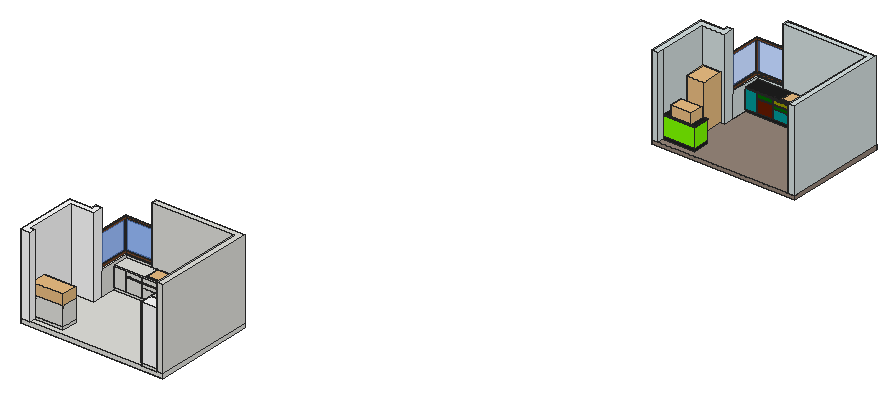
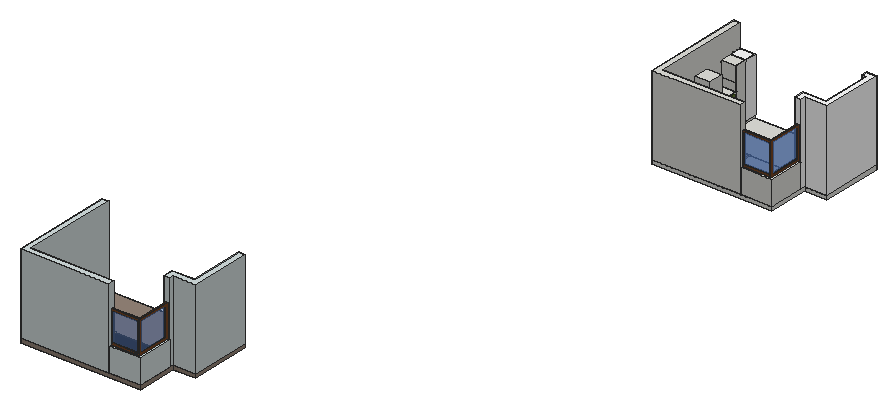
# SketchUp Ruby script. Lengths in inches.
U = 1.inch
M = Sketchup.active_model
def pt(a) = Geom::Point3d.new(a.map { |v| v * U })
def face(e, loops, mat)
  f = e.add_face(loops[0].map { |a| pt(a) })
  loops[1..].each { |l| e.add_face(l.map { |a| pt(a) }).erase! }
  f.material = f.back_material = mat if mat
  f
end
# faces: each face lists its corners as indices into pts; further lists are holes
def faces(e, pts, list, mat = nil) = list.each { |f| face(e, (f[0].is_a?(Array) ? f : [f]).map { |l| l.map { |i| pts[i] } }, mat) }
# xy, xz, yz: faces in a plane at the given z, y or x. An outline is a flat list of corners, or four numbers for a rectangle; further outlines are holes
def ring(l) = l.size == 4 ? [[l[0], l[1]], [l[2], l[1]], [l[2], l[3]], [l[0], l[3]]] : l.each_slice(2).to_a
def flat(e, list, mat, &to3) = list.each { |f| face(e, (f[0].is_a?(Array) ? f : [f]).map { |l| ring(l).map { |u, v| to3.(u, v) } }, mat) }
def xy(e, z, list, mat = nil) = flat(e, list, mat) { |x, y| [x, y, z] }
def xz(e, y, list, mat = nil) = flat(e, list, mat) { |x, z| [x, y, z] }
def yz(e, x, list, mat = nil) = flat(e, list, mat) { |y, z| [x, y, z] }
def lines(e, pts, list) = list.each { |a, b| e.add_line(pt(pts[a]), pt(pts[b])) }
# prism: a flat outline (further loops are holes) pulled along v
def prism(e, loops, v, mat = nil)
  f = face(e, loops, mat); d = Geom::Vector3d.new(v.map { |x| x * U })
  f.pushpull(f.normal.samedirection?(d) ? d.length : -d.length)
end
def box(e, o, s, mat = nil) = prism(e, [[o, [o[0] + s[0], o[1], o[2]], [o[0] + s[0], o[1] + s[1], o[2]], [o[0], o[1] + s[1], o[2]]]], [0, 0, s[2]], mat)
def at(x, y, z, deg = 0) = Geom::Transformation.translation(pt([x, y, z])) * Geom::Transformation.rotation(ORIGIN, Z_AXIS, deg.degrees)
def axes(o, x, y, z) = Geom::Transformation.new([*x, 0, *y, 0, *z, 0, *pt(o).to_a, 1])
def part(name) = M.definitions.add(name)
# library, detail: a bought-in or finely detailed component or shape, given as its bounding box
def library(name, o, s) = part(name).tap { |d| box(d.entities, o, s) }
def detail(e, o, s) = box(e.add_group.entities, o, s)
def put(e, d, t, mat = nil) = e.add_instance(d, t).tap { |i| i.material = mat if mat }
def group(e, t, mat = nil) = e.add_group.tap { |g| g.transformation = t; g.material = mat if mat }.entities
root = M.entities
M.materials.add("Carpaint Yellow 003 1.51cm").color = [255, 255, 255]
M.materials.add("T8600 Mosaic plaster 9142 31.87cm\#1").color = [255, 255, 255]
M.materials.add("[Blacktop New]").color = [30, 30, 30]
M.materials.add("[Carpet Berber Multi]").color = [151, 134, 122]
M.materials.add("[Color B08]").color = [102, 25, 0]
M.materials.add("[Color E07]").color = [153, 153, 0]
M.materials.add("[Color F05]").color = [127, 255, 0]
M.materials.add("[Color G08]").color = [0, 102, 0]
M.materials.add("[Color H07]").color = [0, 153, 153]
M.materials.add("[Translucent Glass Blue]").color = [100, 149, 237]
M.materials["[Translucent Glass Blue]"].alpha = 0.5
M.materials.add("[Translucent Glass Dark Green]").color = [62, 91, 5]
M.materials["[Translucent Glass Dark Green]"].alpha = 0.5
M.materials.add("[Wallpaper Dog Bone]").color = [213, 224, 224]
M.materials.add("[Wood Veneer 01]").color = [120, 70, 37]
c1 = library("Group\#83",[0,0,0],[47.24,22.83,19.96])
c2 = part("OuterShell")
prism(c2.entities,[[[0,0,0.08],[0,0,0.31],[0,0.59,0.31],[0,0.59,0.39],[0,0.79,0.39],[0,0.79,0],[0,0.59,0],[0,0.59,0.08]]],[0.39,0,0])
c3 = part("Cabinet pull handle")
put(c3.entities,c2,at(0,0,0))
put(c3.entities,c2,at(8.62,0,0))
g1 = group(c3.entities,at(0,0,0))
g2 = group(g1,at(0,0,0.2))
xy(g2,0,[[0.39,0.39,8.62,0.79]])
xy(g2,0.12,[[0.39,0.39,8.62,0.59]])
xy(g2,0.2,[[0.39,0.59,8.62,0.63],[0.39,0.63,8.62,0.79]])
xz(g2,0.39,[[0.39,0,8.62,0.12]])
xz(g2,0.59,[[0.39,0.12,8.62,0.2]])
xz(g2,0.79,[[0.39,0,8.62,0.2]])
yz(g2,0.39,[[0.39,0,0.39,0.12,0.59,0.12,0.59,0.2,0.79,0.2,0.79,0]])
yz(g2,8.62,[[0.39,0,0.79,0,0.79,0.2,0.59,0.2,0.59,0.12,0.39,0.12]])
g3 = group(g1,at(0,0,0.2))
xy(g3,-0.2,[[0.39,0.59,8.62,0.63],[0.39,0.63,8.62,0.79]])
xy(g3,-0.12,[[0.39,0.39,8.62,0.59]])
xy(g3,0,[[0.39,0.39,8.62,0.79]])
xz(g3,0.39,[[0.39,-0.12,8.62,0]])
xz(g3,0.59,[[0.39,-0.2,8.62,-0.12]])
xz(g3,0.79,[[0.39,-0.2,8.62,0]])
yz(g3,0.39,[[0.59,-0.2,0.79,-0.2,0.79,0,0.39,0,0.39,-0.12,0.59,-0.12]])
yz(g3,8.62,[[0.59,-0.2,0.59,-0.12,0.39,-0.12,0.39,0,0.79,0,0.79,-0.2]])
c4 = library("1-TABLE DE CUISSON CLC2\#1",[-11.42,-10.04,0],[22.84,20.08,1.26])
c5 = library("Fridge+large\#1",[35.74,-3.43,0],[31.11,25.36,66.28])
c6 = library("3-EVIER M80 CLC2",[-15.18,-9.87,-6.89],[30.32,19.69,21.27])
c7 = library("001",[-50.74,-66.02,15.67],[13.52,1.09,0.48])
c8 = part("Group\#8")
prism(c8.entities,[[[0,0,0],[0,90.79,0],[33.46,90.79,0],[33.46,151.42,0],[210.87,151.42,0],[210.87,0,0]]],[0,0,5.91])
xy(root,0,[[315.4375,884.73,362.68,907.57]])
xy(root,3.9375,[[315.4375,884.73,362.68,907.57]])
xy(root,31.5,[[315.4375,907.57,362.68,908.35]])
xy(root,33.07,[[[315.4375,884.73,362.68,908.35],[341.42,889.22,341.01,889.24,340.61,889.32,340.23,889.46,339.87,889.64,339.53,889.86,339.23,890.13,338.96,890.4375,338.74,890.77,338.56,891.14,338.43,891.52,338.35,891.92,338.32,892.32,338.32,902.2,338.38,902.6,338.5,902.98,338.66,903.35,338.86,903.7,339.11,904.01,339.4,904.29,339.72,904.54,340.07,904.74,340.4375,904.89,340.82,904.99,341.22,905.05,351.3125,905.05,351.68,905.01,352.04,904.93,352.39,904.8,352.72,904.63,353.02,904.43,353.3,904.18,353.55,903.91,353.76,903.6,353.93,903.28,354.0625,902.93,354.15,902.57,354.19,902.2,354.19,892.23,354.17,891.85,354.1,891.48,353.99,891.125,353.83,890.79,353.63,890.47,353.4,890.18,353.125,889.92,352.82,889.69,352.5,889.51,352.15,889.37,351.79,889.27,351.42,889.22],[329.55,889.23,329.21,889.27,328.87,889.34,328.55,889.46,328.24,889.625,327.95,889.82,327.69,890.05,327.46,890.31,327.27,890.59,327.11,890.9,326.99,891.23,326.91,891.5625,326.87,891.91,326.87,902.35,326.91,902.69,326.99,903.03,327.12,903.35,327.28,903.66,327.48,903.94,327.71,904.2,327.98,904.43,328.27,904.62,328.58,904.77,328.91,904.88,329.24,904.95,329.59,904.98,334.5,904.98,334.9,904.92,335.28,904.8,335.65,904.64,335.99,904.4375,336.3,904.1875,336.57,903.9,336.81,903.57,337,903.22,337.14,902.85,337.23,902.46,337.27,902.06,337.27,891.91,337.21,891.57,337.11,891.23,336.97,890.9,336.79,890.59,336.58,890.31,336.33,890.05,336.06,889.82,335.76,889.625,335.44,889.47,335.11,889.35,334.76,889.27,334.41,889.23]]],"[Blacktop New]")
xy(root,36,[[343.16,973.3125,345.66,975.8125],[343.16,975.8125,343.16,1023.93,386.3,1023.93,386.3,1022.68,344.41,1022.68,344.41,975.8125],[344.41,975.8125,344.41,1022.68,386.3,1022.68,386.3,1021.43,345.66,1021.43,345.66,975.8125]])
xy(root,38.5,[[343.16,975.8125,344.41,1021.43],[344.41,975.8125,345.66,1021.43],[345.66,1021.43,383.8,1022.68],[345.66,1022.68,383.8,1023.93]],"[Wood Veneer 01]")
xy(root,81.5,[[343.16,1021.43,345.66,1023.93]])
xy(root,81.5,[[343.16,975.8125,344.41,1021.43],[344.41,975.8125,345.66,1021.43],[345.66,1021.43,383.8,1022.68],[345.66,1022.68,383.8,1023.93]],"[Wood Veneer 01]")
xy(root,84,[[343.16,973.3125,344.41,973.3125,344.41,1022.68,386.3,1022.68,386.3,1023.93,343.16,1023.93],[344.41,973.3125,345.66,973.3125,345.66,1021.43,386.3,1021.43,386.3,1022.68,344.41,1022.68]])
xz(root,884.73,[[315.4375,0,362.68,3.9375],[315.4375,31.5,362.68,33.07]],"[Blacktop New]")
xz(root,884.73,[[315.4375,3.9375,362.68,31.5]],"[Color F05]")
xz(root,907.57,[[315.4375,0,362.68,3.9375]],"[Blacktop New]")
xz(root,907.57,[[315.4375,3.9375,362.68,31.5]],"[Color F05]")
xz(root,908.35,[[315.4375,31.5,362.68,33.07]],"[Blacktop New]")
xz(root,973.3125,[[343.16,36,344.41,84],[344.41,36,345.66,84]])
xz(root,975.8125,[[343.16,36,345.66,38.5]])
xz(root,975.8125,[[343.16,38.5,344.41,81.5],[344.41,38.5,345.66,81.5]],"[Wood Veneer 01]")
xz(root,1021.43,[[343.16,38.5,344.41,81.5]])
xz(root,1021.43,[[345.66,36,386.3,36,386.3,84,345.66,84,345.66,81.5,383.8,81.5,383.8,38.5,345.66,38.5],[344.41,38.5,345.66,81.5]],"[Wood Veneer 01]")
xz(root,1022.68,[[345.66,38.5,383.8,81.5]],"[Translucent Glass Blue]")
xz(root,1023.93,[[[343.16,36,386.3,84],[345.66,38.5,383.8,81.5]]],"[Wood Veneer 01]")
yz(root,315.4375,[[884.73,0,907.57,3.9375],[884.73,31.5,908.35,33.07]])
yz(root,343.16,[[[973.3125,36,1023.93,84],[975.8125,38.5,1021.43,81.5]]],"[Wood Veneer 01]")
yz(root,344.41,[[975.8125,38.5,1021.43,81.5]],"[Translucent Glass Blue]")
yz(root,345.66,[[973.3125,36,1021.43,36,1021.43,38.5,975.8125,38.5,975.8125,81.5,1021.43,81.5,1021.43,84,973.3125,84],[1021.43,38.5,1022.68,81.5],[1022.68,38.5,1023.93,81.5]],"[Wood Veneer 01]")
yz(root,362.68,[[884.73,0,907.57,3.9375],[884.73,31.5,908.35,33.07]],"[Blacktop New]")
yz(root,362.68,[[884.73,3.9375,907.57,31.5]],"[Color F05]")
yz(root,383.8,[[1021.43,38.5,1022.68,81.5],[1022.68,38.5,1023.93,81.5]],"[Wood Veneer 01]")
yz(root,386.3,[[1021.43,36,1022.68,84],[1022.68,36,1023.93,84]])
p = [[348.9,1018.2,31.5],[348.9,1018.2,33.07],[348.9,1018.2,0],[348.9,1018.2,3.9375],[508.35,1018.2,0],[484.73,1018.2,33.07],
  [338.07,895.54,45.01],[338.08,895.48,44.98],[337.87,895.23,44.88],[337.8,895.22,44.88],[337.66,895.25,44.89],[337.61,895.3,44.91],
  [338.07,895.41,44.95],[338.04,895.35,44.93],[338,895.3,44.91],[337.9375,895.25,44.89],[338,895.66,45.05],[338.04,895.61,45.03],
  [337.5625,895.35,44.93],[337.53,895.41,44.95],[337.73,895.73,45.08],[337.8,895.74,45.08],[337.52,895.48,44.98],[337.9375,895.7,45.07],
  [337.73,895.23,44.88],[337.61,895.66,45.05],[337.66,895.7,45.07],[337.87,895.73,45.08],[337.53,895.54,45.01],[337.5625,895.61,45.03]]
lines(root,p,[[0,1],[2,3],[4,2],[5,1],[6,7],[8,9],[10,11],[12,13],[14,15],[7,12],[16,17],[18,19],
  [17,6],[20,21],[19,22],[13,14],[11,18],[23,16],[9,24],[15,8],[24,10],[25,26],[21,27],[22,28],
  [28,29],[29,25],[27,23]])
g4 = group(root,at(0,92.51,0),"Carpaint Yellow 003 1.51cm")
g5 = group(g4,at(0,0,0))
prism(g5,[[[42.44,81.8125,0],[8.98,81.8125,0],[8.98,8.98,0],[14.76,8.98,0],[14.76,0,0],[0,0,0],[0,90.79,0],[33.46,90.79,0],[33.46,97.56,0],[42.44,97.56,0]]],[0,0,118.11])
g6 = group(root,at(8.98,101.49,0))
box(g6,[0,0,0],[47.24,22.83,3.9375])
g7 = group(root,at(8.98,101.49,3.9375))
xy(g7,0,[[0,0,47.24,22.83]])
xz(g7,0,[[0,0,47.24,27.56]])
xz(g7,22.83,[[0,0,47.24,27.56]])
yz(g7,0,[[0,0,22.83,27.56]])
yz(g7,47.24,[[0,0,22.83,27.56]])
put(root,c1,at(8.98,101.49,27.4))
g8 = group(root,at(37.85,192.57,38.58),"[Translucent Glass Blue]")
box(g8,[0,0,0],[0.2,45.62,43])
g9 = group(root,at(42.44,234.95,3.9375))
xy(g9,0,[[0,-22.83,17.72,0]])
xy(g9,0.06,[[0.06,-23.54,17.66,-22.83]])
xy(g9,27.5,[[0.06,-23.54,17.66,-22.83]])
xy(g9,27.56,[[0,-22.83,17.72,0]])
xz(g9,-23.54,[[0.06,0.06,17.66,27.5]])
xz(g9,-22.83,[[[0,0,17.72,27.56],[0.06,0.06,17.66,27.5]]])
xz(g9,0,[[0,0,17.72,27.56]])
yz(g9,0,[[-22.83,0,0,27.56]])
yz(g9,0.06,[[-23.54,0.06,-22.83,27.5]])
yz(g9,17.66,[[-23.54,0.06,-22.83,20.67],[-23.54,20.67,-22.83,27.5]])
yz(g9,17.72,[[-22.83,0,0,20.67],[-22.83,20.67,0,27.56]])
g10 = group(root,at(33.46,190.07,0))
prism(g10,[[[46.38,53.86,0],[46.38,44.88,0],[8.98,44.88,0],[8.98,0,0],[0,0,0],[0,53.86,0]]],[0,0,36.08])
g11 = group(root,at(36.7,190.07,36.08),"[Wood Veneer 01]")
xy(g11,0,[[0,0,0,50.62,43.14,50.62,43.14,48.12,2.5,48.12,2.5,0]])
xy(g11,2.5,[[0,2.5,2.5,48.12],[2.5,48.12,40.64,50.62]])
xy(g11,45.5,[[0,2.5,2.5,48.12],[2.5,48.12,40.64,50.62]])
xy(g11,48,[[0,0,2.5,0,2.5,48.12,43.14,48.12,43.14,50.62,0,50.62]])
xz(g11,0,[[0,0,2.5,48]])
xz(g11,2.5,[[0,2.5,2.5,45.5]])
xz(g11,48.12,[[2.5,0,43.14,0,43.14,48,2.5,48,2.5,45.5,40.64,45.5,40.64,2.5,2.5,2.5],[0,2.5,2.5,45.5]])
xz(g11,50.62,[[[0,0,43.14,48],[2.5,2.5,40.64,45.5]]])
yz(g11,0,[[[0,0,50.62,48],[2.5,2.5,48.12,45.5]]])
yz(g11,2.5,[[0,0,48.12,0,48.12,2.5,2.5,2.5,2.5,45.5,48.12,45.5,48.12,48,0,48],[48.12,2.5,50.62,45.5]])
yz(g11,40.64,[[48.12,2.5,50.62,45.5]])
yz(g11,43.14,[[48.12,0,50.62,48]])
g12 = group(root,at(39.2,239.44,38.58),"[Translucent Glass Blue]")
box(g12,[0,0,0],[38.14,0.2,43])
g13 = group(root,at(60.16,234.95,3.9375))
xy(g13,0,[[0,-22.83,23.62,0]])
xy(g13,0.06,[[0.06,-23.54,23.5625,-22.83]])
xy(g13,19.625,[[0.06,-23.54,23.5625,-22.83]])
xy(g13,20.67,[[0,-22.83,23.62,0]])
xz(g13,-23.54,[[0.06,0.06,23.5625,19.625]])
xz(g13,-22.83,[[[0,0,23.62,20.67],[0.06,0.06,23.5625,19.625]]])
xz(g13,0,[[0,0,23.62,20.67]])
yz(g13,0,[[-22.83,0,0,20.67]])
yz(g13,0.06,[[-23.54,0.06,-22.83,19.625]])
yz(g13,23.5625,[[-23.54,0.06,-22.83,13.78],[-23.54,13.78,-22.83,19.625]])
yz(g13,23.62,[[-22.83,0,0,13.78],[-22.83,13.78,0,20.67]])
g14 = group(root,at(60.16,234.95,24.61))
xy(g14,0,[[0,-22.83,23.62,0]])
xy(g14,0.06,[[0.06,-23.54,23.5625,-22.83]])
xy(g14,6.83,[[0.06,-23.54,23.5625,-22.83]])
xy(g14,6.89,[[0,-22.83,23.62,0]])
xz(g14,-23.54,[[0.06,0.06,23.5625,6.83]])
xz(g14,-22.83,[[[0,0,23.62,6.89],[0.06,0.06,23.5625,6.83]]])
xz(g14,0,[[0,0,23.62,6.89]])
yz(g14,0,[[-22.83,0,0,6.89]])
yz(g14,0.06,[[-23.54,0.06,-22.83,6.83]])
yz(g14,23.5625,[[-23.54,0.06,-22.83,6.83]])
yz(g14,23.62,[[-22.83,0,0,6.89]])
g15 = group(root,at(83.78,234.95,3.9375))
xy(g15,0,[[0,-22.83,35.43,0]])
xy(g15,0.06,[[0.06,-23.54,35.375,-22.83]])
xy(g15,13.72,[[0.06,-23.54,35.375,-22.83]])
xy(g15,13.78,[[0,-22.83,35.43,0]])
xz(g15,-23.54,[[0.06,0.06,35.375,13.72]])
xz(g15,-22.83,[[[0,0,35.43,13.78],[0.06,0.06,35.375,13.72]]])
xz(g15,0,[[0,0,35.43,13.78]])
yz(g15,0,[[-22.83,0,0,13.78]])
yz(g15,0.06,[[-23.54,0.06,-22.83,13.72]])
yz(g15,35.375,[[-23.54,0.06,-22.83,13.72]])
yz(g15,35.43,[[-22.83,0,0,13.78]])
g16 = group(root,at(83.78,234.95,17.72))
xy(g16,0,[[0,-22.83,35.43,0]])
xy(g16,0.06,[[0.06,-23.54,35.375,-22.83]])
xy(g16,5.85,[[0.06,-23.54,35.375,-22.83]])
xy(g16,6.89,[[0,-22.83,35.43,0]])
xz(g16,-23.54,[[0.06,0.06,35.375,5.85]])
xz(g16,-22.83,[[[0,0,35.43,6.89],[0.06,0.06,35.375,5.85]]])
xz(g16,0,[[0,0,35.43,6.89]])
yz(g16,0,[[-22.83,0,0,6.89]])
yz(g16,0.06,[[-23.54,0.06,-22.83,5.85]])
yz(g16,35.375,[[-23.54,0.06,-22.83,5.85]])
yz(g16,35.43,[[-22.83,0,0,6.89]])
g17 = group(root,at(83.78,234.95,24.61))
xy(g17,0,[[0,-22.83,35.43,0]])
xy(g17,0.06,[[0.06,-23.54,35.375,-22.83]])
xy(g17,6.83,[[0.06,-23.54,35.375,-22.83]])
xy(g17,6.89,[[0,-22.83,35.43,0]])
xz(g17,-23.54,[[0.06,0.06,35.375,6.83]])
xz(g17,-22.83,[[[0,0,35.43,6.89],[0.06,0.06,35.375,6.83]]])
xz(g17,0,[[0,0,35.43,6.89]])
yz(g17,0,[[-22.83,0,0,6.89]])
yz(g17,0.06,[[-23.54,0.06,-22.83,6.83]])
yz(g17,35.375,[[-23.54,0.06,-22.83,6.83]])
yz(g17,35.43,[[-22.83,0,0,6.89]])
put(root,c3,axes([60.22,212.12,23.48],[9.17031,0,0],[0,-1,0],[0,0,3]))
put(root,c4,at(102.04,222.98,33.07))
g18 = group(root,at(0,92.51,-6))
prism(g18,[[[33.46,151.42,0],[210.87,151.42,0],[210.87,0,0],[0,0,0],[0,90.79,0],[33.46,90.79,0]]],[0,0,6])
g19 = group(root,at(42.44,234.95,0))
prism(g19,[[[41.34,0,3.9375],[76.77,0,3.9375],[100.39,0,3.9375],[124.02,0,3.9375],[136.61,0,3.9375],[159.45,0,3.9375],[159.45,0,0],[0,0,0],[0,0,3.9375],[17.72,0,3.9375]]],[0,-22.83,0])
g20 = group(root,at(42.44,234.95,31.5))
box(g20,[0,-23.62,0],[159.45,23.62,1.57])
g21 = group(root,at(119.21,234.95,3.9375))
xy(g21,0,[[0,-22.83,23.62,0]])
xy(g21,0.06,[[0.06,-23.54,23.5625,-22.83]])
xy(g21,19.625,[[0.06,-23.54,23.5625,-22.83]])
xy(g21,20.67,[[0,-22.83,23.62,0]])
xz(g21,-23.54,[[0.06,0.06,23.5625,19.625]])
xz(g21,-22.83,[[[0,0,23.62,20.67],[0.06,0.06,23.5625,19.625]]])
xz(g21,0,[[0,0,23.62,20.67]])
yz(g21,0,[[-22.83,0,0,13.78],[-22.83,13.78,0,20.67]])
yz(g21,0.06,[[-23.54,0.06,-22.83,13.78],[-23.54,13.78,-22.83,19.625]])
yz(g21,23.5625,[[-23.54,0.06,-22.83,19.625]])
yz(g21,23.62,[[-22.83,0,0,20.67]])
g22 = group(root,at(119.21,234.95,24.61))
xy(g22,0,[[0,-22.83,23.62,0]])
xy(g22,0.06,[[0.06,-23.54,23.5625,-22.83]])
xy(g22,6.83,[[0.06,-23.54,23.5625,-22.83]])
xy(g22,6.89,[[0,-22.83,23.62,0]])
xz(g22,-23.54,[[0.06,0.06,23.5625,6.83]])
xz(g22,-22.83,[[[0,0,23.62,6.89],[0.06,0.06,23.5625,6.83]]])
xz(g22,0,[[0,0,23.62,6.89]])
yz(g22,0,[[-22.83,0,0,6.89]])
yz(g22,0.06,[[-23.54,0.06,-22.83,6.83]])
yz(g22,23.5625,[[-23.54,0.06,-22.83,6.83]])
yz(g22,23.62,[[-22.83,0,0,6.89]])
g23 = group(root,at(79.84,92.51,0))
g24 = group(g23,at(0,0,0))
prism(g24,[[[131.02,0,0],[122.05,0,0],[122.05,142.44,0],[0,142.44,0],[0,151.42,0],[131.02,151.42,0]]],[0,0,118.11])
g25 = group(root,at(142.83,234.95,3.9375))
xy(g25,0,[[0,-22.83,23.62,0]])
xy(g25,0.06,[[0.06,-23.54,23.5625,-22.83]])
xy(g25,27.5,[[0.06,-23.54,23.5625,-22.83]])
xy(g25,27.56,[[0,-22.83,23.62,0]])
xz(g25,-23.54,[[0.06,0.06,23.5625,27.5]])
xz(g25,-22.83,[[[0,0,23.62,27.56],[0.06,0.06,23.5625,27.5]]])
xz(g25,0,[[0,0,23.62,27.56]])
yz(g25,0,[[-22.83,0,0,20.67],[-22.83,20.67,0,27.56]])
yz(g25,0.06,[[-23.54,0.06,-22.83,27.5]])
yz(g25,23.5625,[[-23.54,0.06,-22.83,27.5]])
yz(g25,23.62,[[-22.83,0,0,27.56]])
g26 = group(root,at(166.46,234.95,3.9375))
xy(g26,0,[[0,-22.83,12.6,0]])
xy(g26,0.06,[[0.06,-23.54,10.96,-22.83]])
xy(g26,27.5,[[0.06,-23.54,10.96,-22.83]])
xy(g26,27.56,[[0,-22.83,12.6,0]])
xz(g26,-23.54,[[0.06,0.06,10.96,27.5]])
xz(g26,-22.83,[[[0,0,12.6,27.56],[0.06,0.06,12.54,27.5]],[10.96,0.06,11.02,27.5],[11.02,0.06,12.54,27.5]])
xz(g26,0,[[0,0,12.6,27.56]])
yz(g26,0,[[-22.83,0,0,27.56]])
yz(g26,0.06,[[-23.54,0.06,-22.83,27.5]])
yz(g26,10.96,[[-23.54,0.06,-22.83,27.5]])
yz(g26,12.6,[[-22.83,0,0,27.56]])
g27 = group(root,at(201.89,234.95,31.5))
prism(g27,[[[-23.62,-22.83,0],[-23.62,-35.43,0],[-23.62,-61.02,0],[-23.62,-81.42,0],[-23.62,-81.42,1.57],[-23.62,-57.8,1.57],[-23.62,0,1.57],[-23.62,0,0]]],[23.62,0,0])
g28 = group(root,at(201.89,153.54,3.9375))
xy(g28,0,[[-22.83,-25.59,0,0]])
xy(g28,0.06,[[-23.54,-25.53,-22.83,-0.06]])
xy(g28,22.22,[[-23.54,-25.53,-22.83,-0.06]])
xy(g28,22.28,[[-22.83,-25.59,0,0]])
xz(g28,-25.59,[[-22.83,0,0,22.28]])
xz(g28,-25.53,[[-23.54,0.06,-22.83,22.22]])
xz(g28,-0.06,[[-23.54,0.06,-22.83,22.22]])
xz(g28,0,[[-22.83,0,0,22.28]])
yz(g28,-23.54,[[-25.53,0.06,-0.06,22.22]])
yz(g28,-22.83,[[[-25.59,0,0,22.28],[-25.53,0.06,-0.06,22.22]]])
yz(g28,0,[[-25.59,0,0,22.28]])
g29 = group(root,at(201.89,199.52,3.9375))
xy(g29,0,[[-22.83,-25.59,0,0]])
xy(g29,0.06,[[-23.54,-25.53,-22.83,-0.06]])
xy(g29,13.72,[[-23.54,-25.53,-22.83,-0.06]])
xy(g29,13.78,[[-22.83,-25.59,0,0]])
xz(g29,-25.59,[[-22.83,0,0,13.78]])
xz(g29,-25.53,[[-23.54,0.06,-22.83,13.72]])
xz(g29,-0.06,[[-23.54,0.06,-22.83,13.72]])
xz(g29,0,[[-22.83,0,0,13.78]])
yz(g29,-23.54,[[-25.53,0.06,-0.06,13.72]])
yz(g29,-22.83,[[[-25.59,0,0,13.78],[-25.53,0.06,-0.06,13.72]]])
yz(g29,0,[[-25.59,0,0,13.78]])
g30 = group(root,at(201.89,173.93,3.9375))
xy(g30,0,[[-22.83,-20.39,0,-17.72],[-22.83,-17.72,0,0]])
xy(g30,0.06,[[-23.54,-20.33,-22.83,-0.06]])
xy(g30,27.5,[[-23.54,-20.33,-22.83,-0.06]])
xy(g30,27.56,[[-22.83,-20.39,0,0]])
xz(g30,-20.39,[[-22.83,0,0,22.28],[-22.83,22.28,0,27.56]])
xz(g30,-20.33,[[-23.54,0.06,-22.83,22.28],[-23.54,22.28,-22.83,27.5]])
xz(g30,-0.06,[[-23.54,0.06,-22.83,27.5]])
xz(g30,0,[[-22.83,0,0,13.78],[-22.83,13.78,0,27.56]])
yz(g30,-23.54,[[-20.33,0.06,-0.06,27.5]])
yz(g30,-22.83,[[[-20.39,0,0,27.56],[-20.33,0.06,-0.06,27.5]]])
yz(g30,0,[[-20.39,0,0,27.56]])
g31 = group(root,at(201.89,127.95,3.9375))
xy(g31,0,[[-22.83,-17.72,0,0]])
xy(g31,0.06,[[-23.54,-17.66,-22.83,-0.06]])
xy(g31,80.26,[[-23.54,-17.66,-22.83,-0.06]])
xy(g31,80.31,[[-22.83,-17.72,0,0]])
xz(g31,-17.72,[[-22.83,0,0,80.31]])
xz(g31,-17.66,[[-23.54,0.06,-22.83,80.26]])
xz(g31,-0.06,[[-23.54,0.06,-22.83,22.28],[-23.54,22.28,-22.83,45.91],[-23.54,45.91,-22.83,58.03],[-23.54,58.03,-22.83,80.26]])
xz(g31,0,[[-22.83,0,0,22.28],[-22.83,22.28,0,45.91],[-22.83,45.91,0,58.03],[-22.83,58.03,0,80.31]])
yz(g31,-23.54,[[-17.66,0.06,-0.06,80.26]])
yz(g31,-22.83,[[[-17.72,0,0,80.31],[-17.66,0.06,-0.06,80.26]]])
yz(g31,0,[[-17.72,0,0,80.31]])
g32 = group(root,at(201.89,110.23,3.9375),"T8600 Mosaic plaster 9142 31.87cm\#1")
xy(g32,0,[[-22.83,-17.72,0,0]])
xy(g32,0.06,[[-23.54,-17.66,-22.83,-0.06]])
xy(g32,80.26,[[-23.54,-17.66,-22.83,-0.06]])
xy(g32,80.31,[[-22.83,-17.72,0,0]])
xz(g32,-17.72,[[-22.83,0,0,80.31]])
xz(g32,-17.66,[[-23.54,0.06,-22.83,80.26]])
xz(g32,-0.06,[[-23.54,0.06,-22.83,80.26]])
xz(g32,0,[[-22.83,0,0,80.31]])
yz(g32,-23.54,[[-17.66,0.06,-0.06,80.26]])
yz(g32,-22.83,[[[-17.72,0,0,80.31],[-17.66,0.06,-0.06,80.26]]])
yz(g32,0,[[-17.72,0,0,80.31]])
g33 = group(root,at(201.89,212.12,3.9375))
xy(g33,0,[[-22.83,-12.6,0,0]])
xy(g33,0.06,[[-23.54,-12.54,-22.83,-1.63]])
xy(g33,27.5,[[-23.54,-12.54,-22.83,-1.63]])
xy(g33,27.56,[[-22.83,-12.6,0,0]])
xz(g33,-12.6,[[-22.83,0,0,13.78],[-22.83,13.78,0,27.56]])
xz(g33,-12.54,[[-23.54,0.06,-22.83,13.78],[-23.54,13.78,-22.83,27.5]])
xz(g33,-1.63,[[-23.54,0.06,-22.83,27.5]])
xz(g33,0,[[-22.83,0,0,27.56]])
yz(g33,-23.54,[[-12.54,0.06,-1.63,27.5]])
yz(g33,-22.83,[[[-12.6,0,0,27.56],[-12.54,0.06,-0.06,27.5]],[-1.63,0.06,-1.57,27.5],[-1.57,0.06,-0.06,27.5]])
yz(g33,0,[[-12.6,0,0,27.56]])
g34 = group(root,at(201.89,199.52,17.72))
xy(g34,0,[[-22.83,-25.59,0,0]])
xy(g34,0.06,[[-23.54,-25.53,-22.83,-0.06]])
xy(g34,13.72,[[-23.54,-25.53,-22.83,-0.06]])
xy(g34,13.78,[[-22.83,-25.59,0,0]])
xz(g34,-25.59,[[-22.83,0,0,13.78]])
xz(g34,-25.53,[[-23.54,0.06,-22.83,13.72]])
xz(g34,-0.06,[[-23.54,0.06,-22.83,13.72]])
xz(g34,0,[[-22.83,0,0,13.78]])
yz(g34,-23.54,[[-25.53,0.06,-0.06,13.72]])
yz(g34,-22.83,[[[-25.59,0,0,13.78],[-25.53,0.06,-0.06,13.72]]])
yz(g34,0,[[-25.59,0,0,13.78]])
g35 = group(root,at(201.89,153.54,26.22))
xy(g35,0,[[-23.54,-25.59,-22.83,0],[-22.83,-25.59,0,0]])
xy(g35,0.71,[[-23.54,-24.88,-23.39,-0.71],[-23.39,-24.88,-23.1875,-0.71],[-23.1875,-24.88,-22.83,-0.71],[-22.83,-24.88,-0.71,-0.71]])
xy(g35,22.91,[[-23.54,-24.88,-23.39,-0.71],[-23.39,-24.88,-23.1875,-0.71],[-23.1875,-24.88,-22.83,-0.71],[-22.83,-24.88,-0.71,-0.71]])
xy(g35,23.62,[[-23.54,-25.59,-22.83,0],[-22.83,-25.59,0,0]])
xz(g35,-25.59,[[-23.54,0,-22.83,23.62],[-22.83,0,0,23.62]])
xz(g35,-24.88,[[-23.54,0.71,-23.39,22.91],[-23.39,0.71,-23.1875,22.91],[-23.1875,0.71,-22.83,22.91],[-22.83,0.71,-0.71,22.91]])
xz(g35,-0.71,[[-23.54,0.71,-23.39,22.91],[-23.39,0.71,-23.1875,22.91],[-23.1875,0.71,-22.83,22.91],[-22.83,0.71,-0.71,22.91]])
xz(g35,0,[[-23.54,0,-22.83,5.28],[-22.83,0,0,5.28],[-23.54,5.28,-22.83,6.85],[-22.83,5.28,0,6.85],[-23.54,6.85,-22.83,23.62],
  [-22.83,6.85,0,23.62]])
yz(g35,-23.54,[[[-25.59,0,0,23.62],[-24.88,0.71,-0.71,22.91]]])
yz(g35,-23.39,[[-24.88,0.71,-0.71,22.91]],"[Translucent Glass Dark Green]")
yz(g35,-23.1875,[[-24.88,0.71,-0.71,22.91]],"[Translucent Glass Dark Green]")
yz(g35,-22.83,[[[-25.59,0,0,23.62],[-24.88,0.71,-0.71,22.91]]])
yz(g35,-0.71,[[-24.88,0.71,-0.71,22.91]])
yz(g35,0,[[-25.59,0,0,23.62]])
g36 = group(root,at(201.89,234.95,3.9375))
box(g36,[-22.83,-22.83,0],[22.83,22.83,27.56])
g37 = group(root,at(201.89,234.95,0))
prism(g37,[[[-22.83,-81.42,3.9375],[-22.83,-78.74,3.9375],[-22.83,-61.02,3.9375],[-22.83,-35.43,3.9375],[-22.83,-22.83,3.9375],[-22.83,0,3.9375],[-22.83,0,0],[-22.83,-142.44,0],[-22.83,-142.44,3.9375],[-22.83,-124.72,3.9375],[-22.83,-107.01,3.9375]]],[22.83,0,0])
g38 = group(root,at(201.89,177.16,33.07))
prism(g38,[[[-22.83,0,51.18],[-22.83,0,0],[-22.83,-23.62,0],[-22.83,-23.62,16.77],[-22.83,-23.62,28.9],[-22.83,-23.62,51.18]]],[22.83,0,0])
put(root,c5,at(339.37,890.59,0,90))
put(root,c6,axes([340.47,897.08,33.09],[1,0,0],[0,-1,0],[0,0,1]))
g39 = group(root,at(348.9,1018.2,3.9375),"[Color H07]")
xy(g39,0,[[0,-22.83,17.72,0]])
xy(g39,0.06,[[0.06,-23.54,17.66,-22.83]])
xy(g39,27.5,[[0.06,-23.54,17.66,-22.83]])
xy(g39,27.56,[[0,-22.83,17.72,0]])
xz(g39,-23.54,[[0.06,0.06,17.66,27.5]])
xz(g39,-22.83,[[[0,0,17.72,27.56],[0.06,0.06,17.66,27.5]]])
xz(g39,0,[[0,0,17.72,27.56]])
yz(g39,0,[[-22.83,0,0,27.56]])
yz(g39,0.06,[[-23.54,0.06,-22.83,27.5]])
yz(g39,17.66,[[-23.54,0.06,-22.83,20.67],[-23.54,20.67,-22.83,27.5]])
yz(g39,17.72,[[-22.83,0,0,20.67],[-22.83,20.67,0,27.56]])
g40 = group(root,at(339.92,973.3125,0),"[Wallpaper Dog Bone]")
prism(g40,[[[0,53.86,0],[46.38,53.86,0],[46.38,44.88,0],[8.98,44.88,0],[8.98,0,0],[0,0,0]]],[0,0,36])
g41 = group(root,at(366.62,1018.2,3.9375),"[Color B08]")
xy(g41,0,[[0,-22.83,23.62,0]])
xy(g41,0.06,[[0.06,-23.54,23.5625,-22.83]])
xy(g41,19.625,[[0.06,-23.54,23.5625,-22.83]])
xy(g41,20.67,[[0,-22.83,23.62,0]])
xz(g41,-23.54,[[0.06,0.06,23.5625,19.625]])
xz(g41,-22.83,[[[0,0,23.62,20.67],[0.06,0.06,23.5625,19.625]]])
xz(g41,0,[[0,0,23.62,20.67]])
yz(g41,0,[[-22.83,0,0,20.67]])
yz(g41,0.06,[[-23.54,0.06,-22.83,19.625]])
yz(g41,23.5625,[[-23.54,0.06,-22.83,13.78],[-23.54,13.78,-22.83,19.625]])
yz(g41,23.62,[[-22.83,0,0,13.78],[-22.83,13.78,0,20.67]])
g42 = group(root,at(366.62,1018.2,24.61),"[Color G08]")
xy(g42,0,[[0,-22.83,23.62,0]])
xy(g42,0.06,[[0.06,-23.54,23.5625,-22.83]])
xy(g42,5.85,[[0.06,-23.54,23.5625,-22.83]])
xy(g42,6.89,[[0,-22.83,23.62,0]])
xz(g42,-23.54,[[0.06,0.06,23.5625,5.85]])
xz(g42,-22.83,[[[0,0,23.62,6.89],[0.06,0.06,23.5625,5.85]]])
xz(g42,0,[[0,0,23.62,6.89]])
yz(g42,0,[[-22.83,0,0,6.89]])
yz(g42,0.06,[[-23.54,0.06,-22.83,5.85]])
yz(g42,23.5625,[[-23.54,0.06,-22.83,5.85]])
yz(g42,23.62,[[-22.83,0,0,6.89]])
put(root,c7,axes([588.1875,1060.31,7.89],[4.36782,0,0],[0,1,0],[0,0,1]))
g43 = group(root,at(390.24,1018.2,3.9375),"[Color H07]")
xy(g43,0,[[0,-22.83,35.43,0]])
xy(g43,0.06,[[0.06,-23.54,35.375,-22.83]])
xy(g43,13.72,[[0.06,-23.54,35.375,-22.83]])
xy(g43,13.78,[[0,-22.83,35.43,0]])
xz(g43,-23.54,[[0.06,0.06,35.375,13.72]])
xz(g43,-22.83,[[[0,0,35.43,13.78],[0.06,0.06,35.375,13.72]]])
xz(g43,0,[[0,0,35.43,13.78]])
yz(g43,0,[[-22.83,0,0,13.78]])
yz(g43,0.06,[[-23.54,0.06,-22.83,13.72]])
yz(g43,35.375,[[-23.54,0.06,-22.83,13.72]])
yz(g43,35.43,[[-22.83,0,0,13.78]])
g44 = group(root,at(390.24,1018.2,17.72),"[Color G08]")
xy(g44,0,[[0,-22.83,35.43,0]])
xy(g44,0.06,[[0.06,-23.54,35.375,-22.83]])
xy(g44,5.85,[[0.06,-23.54,35.375,-22.83]])
xy(g44,6.89,[[0,-22.83,35.43,0]])
xz(g44,-23.54,[[0.06,0.06,35.375,5.85]])
xz(g44,-22.83,[[[0,0,35.43,6.89],[0.06,0.06,35.375,5.85]]])
xz(g44,0,[[0,0,35.43,6.89]])
yz(g44,0,[[-22.83,0,0,6.89]])
yz(g44,0.06,[[-23.54,0.06,-22.83,5.85]])
yz(g44,35.375,[[-23.54,0.06,-22.83,5.85]])
yz(g44,35.43,[[-22.83,0,0,6.89]])
g45 = group(root,at(390.24,1018.2,24.61),"[Color E07]")
xy(g45,0,[[0,-22.83,35.43,0]])
xy(g45,0.06,[[0.06,-23.54,35.375,-22.83]])
xy(g45,5.85,[[0.06,-23.54,35.375,-22.83]])
xy(g45,6.89,[[0,-22.83,35.43,0]])
xz(g45,-23.54,[[0.06,0.06,35.375,5.85]])
xz(g45,-22.83,[[[0,0,35.43,6.89],[0.06,0.06,35.375,5.85]]])
xz(g45,0,[[0,0,35.43,6.89]])
yz(g45,0,[[-22.83,0,0,6.89]])
yz(g45,0.06,[[-23.54,0.06,-22.83,5.85]])
yz(g45,35.375,[[-23.54,0.06,-22.83,5.85]])
yz(g45,35.43,[[-22.83,0,0,6.89]])
put(root,c8,at(306.46,875.75,-5.91),"[Carpet Berber Multi]")
g46 = group(root,at(306.46,875.75,0),"[Wallpaper Dog Bone]")
p = [[33.46,151.42,0],[33.46,97.56,0],[60.16,0,0],[201.89,0,0],[42.44,142.44,0],[42.44,97.56,0],
  [79.84,151.42,0],[79.84,142.44,0]]
lines(g46,p,[[0,1],[2,3],[4,5],[6,0],[7,4]])
g47 = group(g46,at(0,0,0))
g48 = group(g47,at(0,0,0))
prism(g48,[[[0,0,0],[0,90.79,0],[33.46,90.79,0],[33.46,97.56,0],[42.44,97.56,0],[42.44,81.8125,0],[8.98,81.8125,0],[8.98,8.98,0],[9.49,8.98,0],[9.49,0,0]]],[0,0,118.11])
g49 = group(g46,at(79.84,0,0))
g50 = group(g49,at(0,0,0))
prism(g50,[[[0,151.42,0],[131.02,151.42,0],[131.02,0,0],[122.05,0,0],[122.05,142.44,0],[0,142.44,0]]],[0,0,118.11])
put(root,c4,at(413.24,1005.83,33.07))
put(root,c7,axes([806.86,1060.31,14.78],[8.6774,0,0],[0,1,0],[0,0,1]))
g51 = group(root,at(348.9,995.36,0),"[Blacktop New]")
box(g51,[0,0,0],[159.45,22.83,3.9375])
g52 = group(root,at(348.9,1018.2,31.5),"[Blacktop New]")
box(g52,[0,-23.62,0],[159.45,23.62,1.57])
g53 = group(root,at(425.67,1018.2,3.9375),"[Color B08]")
xy(g53,0,[[0,-22.83,23.62,0]])
xy(g53,0.06,[[0.06,-23.54,23.5625,-22.83]])
xy(g53,20.61,[[0.06,-23.54,23.5625,-22.83]])
xy(g53,20.67,[[0,-22.83,23.62,0]])
xz(g53,-23.54,[[0.06,0.06,23.5625,20.61]])
xz(g53,-22.83,[[[0,0,23.62,20.67],[0.06,0.06,23.5625,20.61]]])
xz(g53,0,[[0,0,23.62,20.67]])
yz(g53,0,[[-22.83,0,0,13.78],[-22.83,13.78,0,20.67]])
yz(g53,0.06,[[-23.54,0.06,-22.83,13.78],[-23.54,13.78,-22.83,20.61]])
yz(g53,23.5625,[[-23.54,0.06,-22.83,20.61]])
yz(g53,23.62,[[-22.83,0,0,20.67]])
g54 = group(root,at(425.67,1018.2,24.61),"[Color G08]")
xy(g54,0,[[0,-22.83,23.62,0]])
xy(g54,0.06,[[0.06,-23.54,23.5625,-22.83]])
xy(g54,5.85,[[0.06,-23.54,23.5625,-22.83]])
xy(g54,6.89,[[0,-22.83,23.62,0]])
xz(g54,-23.54,[[0.06,0.06,23.5625,5.85]])
xz(g54,-22.83,[[[0,0,23.62,6.89],[0.06,0.06,23.5625,5.85]]])
xz(g54,0,[[0,0,23.62,6.89]])
yz(g54,0,[[-22.83,0,0,6.89]])
yz(g54,0.06,[[-23.54,0.06,-22.83,5.85]])
yz(g54,23.5625,[[-23.54,0.06,-22.83,5.85]])
yz(g54,23.62,[[-22.83,0,0,6.89]])
